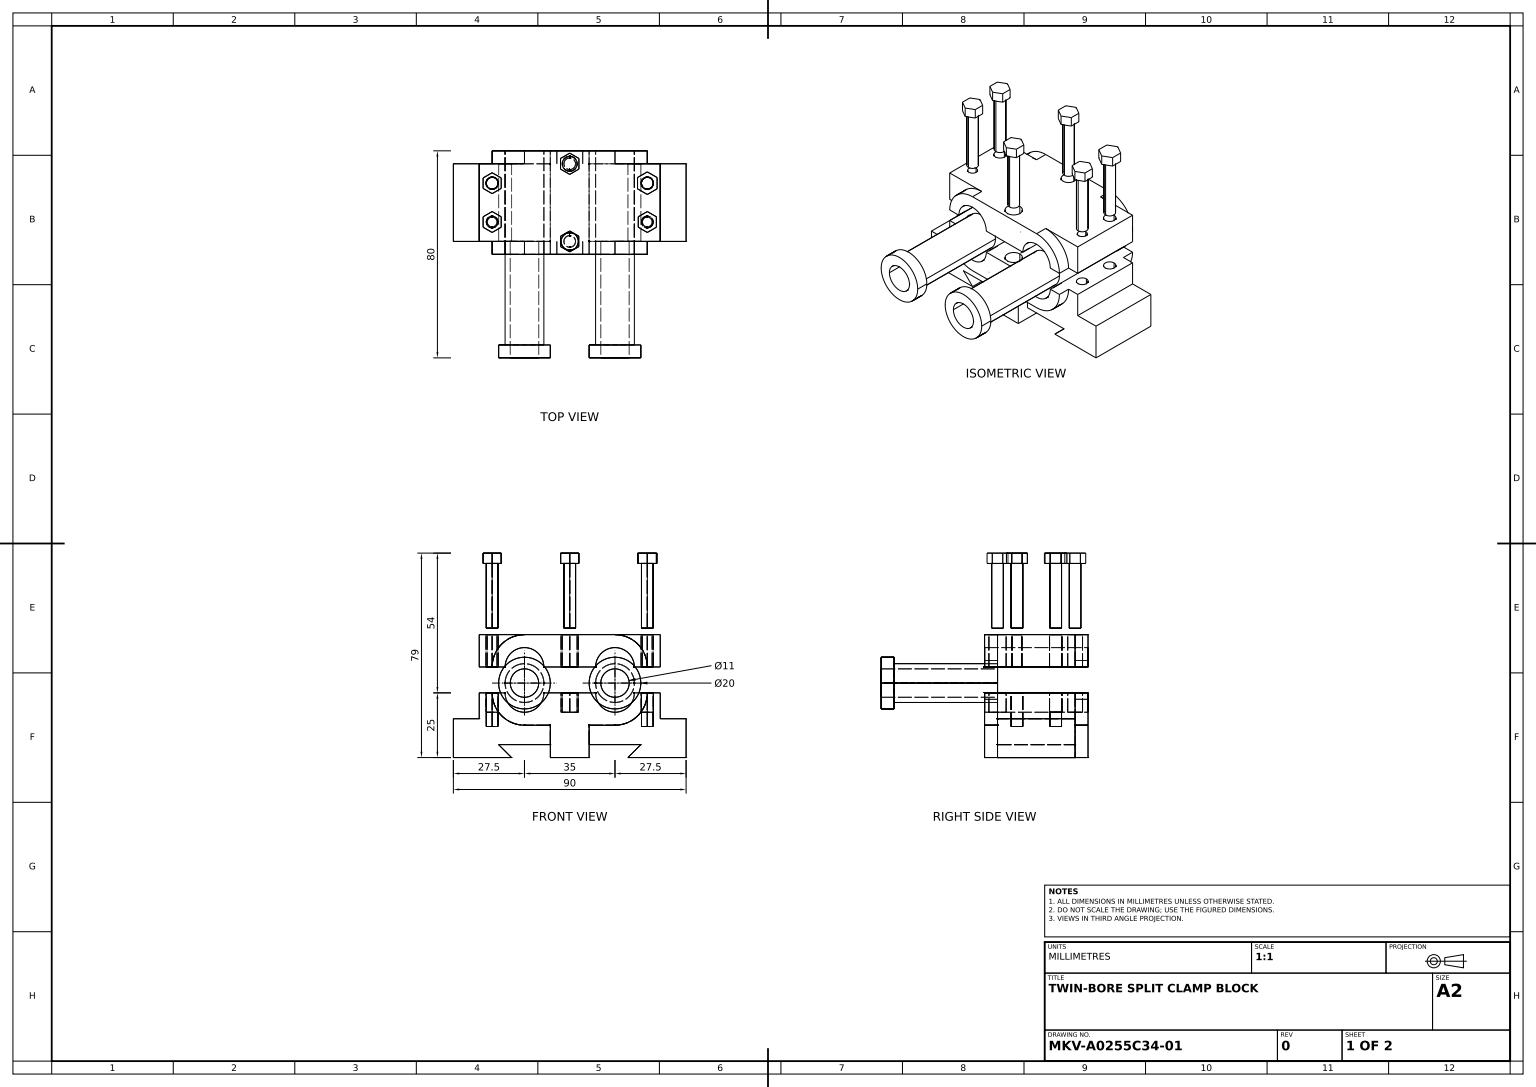
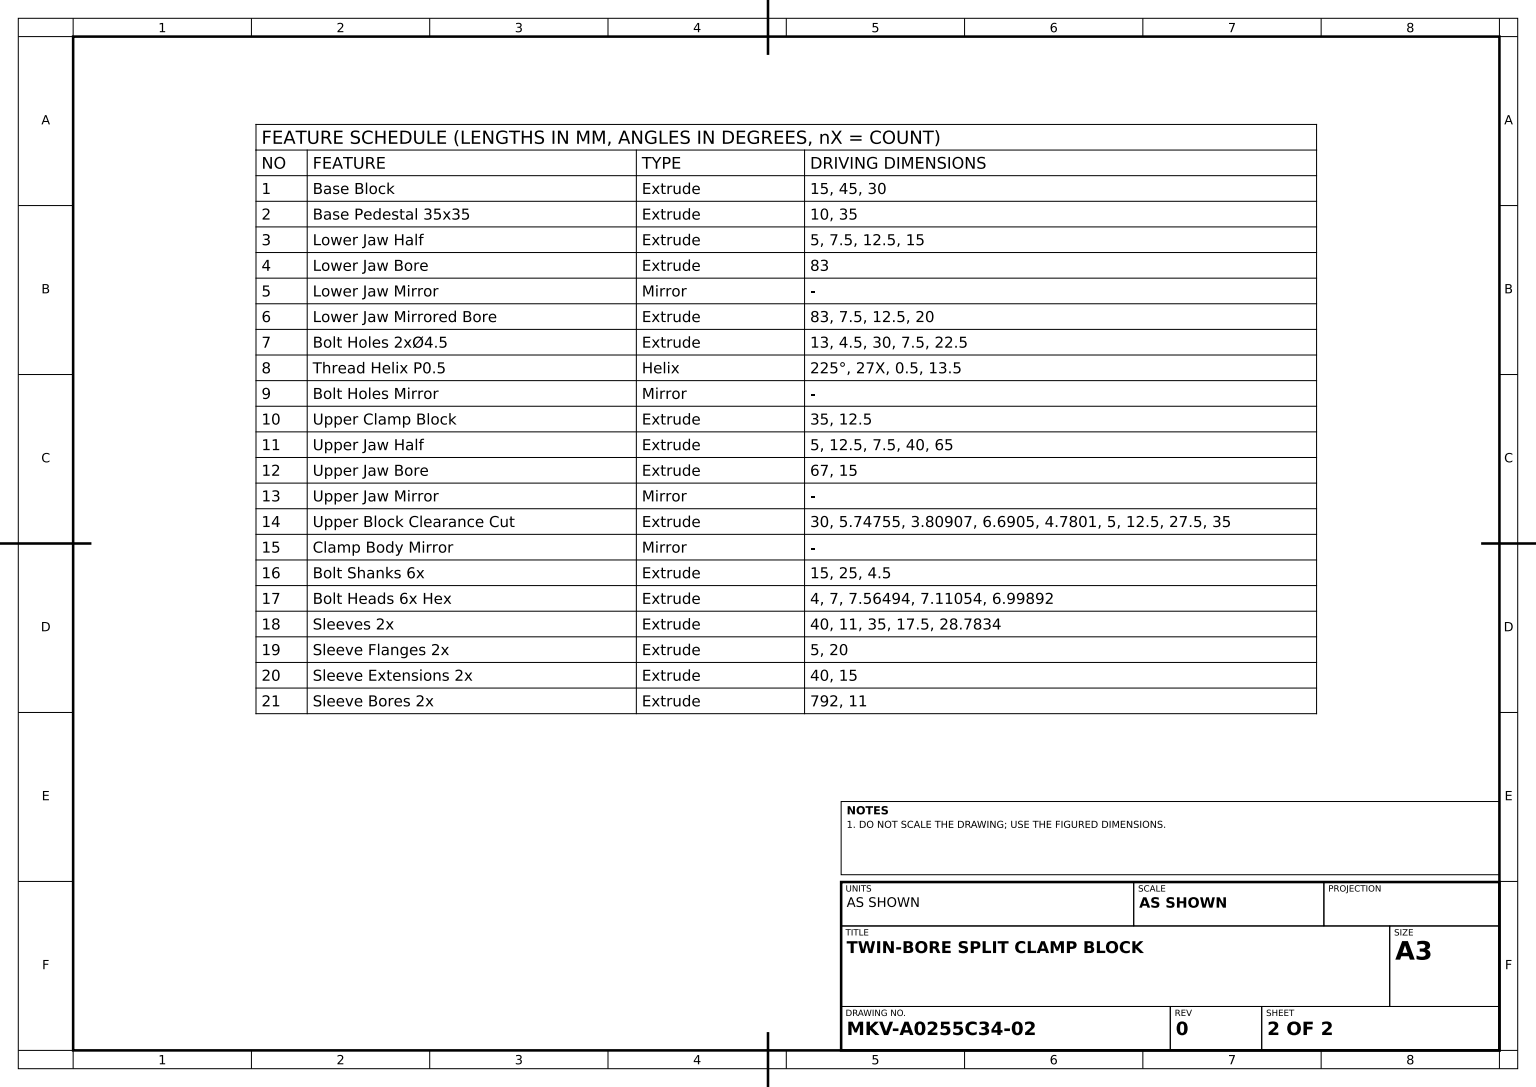
solid
v1 (-7.5,0,5)
v2 (-7.5,12.5,5)
e1 v1 v2 LINE
v3 (-7.5,12.5,0)
e2 v2 v3 LINE
v4 (-7.5,5,0)
e3 v4 v3 LINE
v5 (-7.5,5,-30)
e4 v4 v5 LINE
v6 (-7.5,12.5,-30)
e5 v5 v6 LINE
v7 (-7.5,12.5,-35)
e6 v7 v6 LINE
v8 (-7.5,0,-35)
e7 v8 v7 LINE
e8 v1 v8 LINE
face PLANE(AX(P(-7.5,0,5),D(-1,0,0),D(0,0,1))) [e1 e2 -e3 e4 e5 -e6 -e7 -e8]
v9 (35,15,0)
v10 (35,15,-30)
e9 v9 v10 LINE
v11 (35,25,-30)
e10 v11 v10 LINE
v12 (35,25,0)
e11 v12 v11 LINE
e12 v12 v9 LINE
face PLANE(AX(P(35,25,-30),D(-1,0,0),D(0,0,1))) rev [e9 -e10 -e11 e12]
v13 (-30,25,-20.109948)
v14 (-30,25,-24.890052)
e13 v13 v14 CIRCLE(AX(P(-30,25,-22.5),D(0,1,0),D(0,0,-1)),2.390052)
e14 v14 v13 CIRCLE(AX(P(-30,25,-22.5),D(0,1,0),D(0,0,-1)),2.390052)
v15 (-30,25,-9.75)
v16 (-30,25,-5.25)
e15 v15 v16 CIRCLE(AX(P(-30,25,-7.5),D(0,-1,0),D(0,0,1)),2.25)
e16 v16 v15 CIRCLE(AX(P(-30,25,-7.5),D(0,-1,0),D(0,0,1)),2.25)
v17 (-35,25,0)
v18 (-30,25,0)
e17 v17 v18 LINE
v19 (-30,25,5)
e18 v19 v18 LINE
v20 (-25,25,5)
e19 v20 v19 LINE
v21 (-25,25,-35)
e20 v20 v21 LINE
v22 (-30,25,-35)
e21 v21 v22 LINE
v23 (-30,25,-30)
e22 v22 v23 LINE
v24 (-35,25,-30)
e23 v23 v24 LINE
e24 v24 v17 LINE
face PLANE(AX(P(0,25,0),D(0,-1,0),D(0,0,-1))) rev [-e13 -e14] [e15 e16] [e17 -e18 -e19 e20 e21 e22 e23 e24]
v25 (30,25,-20.109948)
v26 (30,25,-24.890052)
e25 v25 v26 CIRCLE(AX(P(30,25,-22.5),D(0,-1,0),D(0,0,-1)),2.390052)
v27 (30,17.5,-20.109948)
e26 v27 v25 LINE
v28 (30,17.5,-24.890052)
e27 v28 v27 CIRCLE(AX(P(30,17.5,-22.5),D(0,1,0),D(0,0,1)),2.390052)
e28 v28 v26 LINE
face CYL(AX(P(30,17.5,-22.5),D(0,1,0),D(0,0,1)),2.390052) rev [-e25 -e26 -e27 e28]
v29 (0,17.5,3.345252)
v30 (0,25,3.345252)
e29 v29 v30 LINE
v31 (0,25,-3.345252)
e30 v31 v30 CIRCLE(AX(P(0,25,0),D(0,-1,0),D(0,0,-1)),3.345252)
v32 (0,17.5,-3.345252)
e31 v32 v31 LINE
e32 v29 v32 CIRCLE(AX(P(0,17.5,0),D(0,1,0),D(0,0,1)),3.345252)
face CYL(AX(P(0,17.5,0),D(0,1,0),D(0,0,1)),3.345252) rev [e29 -e30 -e31 -e32]
v33 (0,17.5,-32.873773)
v34 (0,25,-32.873773)
e33 v33 v34 LINE
v35 (0,17.5,-27.126227)
e34 v35 v33 CIRCLE(AX(P(0,17.5,-30),D(0,1,0),D(0,0,1)),2.873773)
v36 (0,25,-27.126227)
e35 v35 v36 LINE
e36 v34 v36 CIRCLE(AX(P(0,25,-30),D(0,-1,0),D(0,0,-1)),2.873773)
face CYL(AX(P(0,17.5,-30),D(0,1,0),D(0,0,1)),2.873773) rev [-e33 -e34 e35 -e36]
e37 v32 v29 CIRCLE(AX(P(0,17.5,0),D(0,1,0),D(0,0,1)),3.345252)
e38 v30 v31 CIRCLE(AX(P(0,25,0),D(0,-1,0),D(0,0,-1)),3.345252)
face CYL(AX(P(0,17.5,0),D(0,1,0),D(0,0,1)),3.345252) rev [-e37 e31 -e38 -e29]
v37 (-30,12,-5.25)
v38 (-30,12,-9.75)
e39 v37 v38 CIRCLE(AX(P(-30,12,-7.5),D(0,-1,0),D(0,0,1)),2.25)
e40 v38 v37 CIRCLE(AX(P(-30,12,-7.5),D(0,-1,0),D(0,0,1)),2.25)
face PLANE(AX(P(-30,12,-7.5),D(0,1,0),D(0,0,1))) [-e39 -e40]
v39 (30,12,-5.25)
v40 (30,25,-5.25)
e41 v39 v40 LINE
v41 (30,12,-9.75)
e42 v41 v39 CIRCLE(AX(P(30,12,-7.5),D(0,1,0),D(0,0,1)),2.25)
v42 (30,25,-9.75)
e43 v41 v42 LINE
e44 v42 v40 CIRCLE(AX(P(30,25,-7.5),D(0,1,0),D(0,0,1)),2.25)
face CYL(AX(P(30,12,-7.5),D(0,1,0),D(0,0,1)),2.25) rev [-e41 -e42 e43 e44]
face PLANE(AX(P(0,17.5,0),D(0,1,0),D(0,0,1))) [e37 e32]
v43 (45,0,-30)
v44 (22.5,0,-30)
e45 v43 v44 LINE
v45 (45,0,0)
e46 v45 v43 LINE
v46 (22.5,0,0)
e47 v46 v45 LINE
e48 v46 v44 LINE
face PLANE(AX(P(0,0,0),D(0,-1,0),D(0,0,-1))) [-e45 -e46 -e47 e48]
v47 (17.5,12.5,-35)
v48 (17.5,12.5,-30)
e49 v47 v48 LINE
v49 (30,25,-35)
e50 v47 v49 CIRCLE(AX(P(17.5,25,-35),D(0,0,1),D(1,0,0)),12.5)
v50 (30,25,-30)
e51 v49 v50 LINE
e52 v48 v50 CIRCLE(AX(P(17.5,25,-30),D(0,0,1),D(1,0,0)),12.5)
face CYL(AX(P(17.5,25,-35),D(0,0,1),D(1,0,0)),12.5) [-e49 e50 e51 -e52]
v51 (-17.5,12.5,0)
e53 v3 v51 LINE
v52 (-17.5,12.5,5)
e54 v2 v52 LINE
e55 v52 v51 LINE
face PLANE(AX(P(0,12.5,5),D(0,-1,0),D(0,0,-1))) [-e53 -e2 e54 e55]
v53 (7.5,0,-35)
e56 v8 v53 LINE
v54 (7.5,0,5)
e57 v54 v53 LINE
e58 v1 v54 LINE
face PLANE(AX(P(0,0,0),D(0,-1,0),D(0,0,-1))) [e8 e56 -e57 -e58]
v55 (30,12,-20.25)
v56 (30,12,-24.75)
e59 v55 v56 CIRCLE(AX(P(30,12,-22.5),D(0,1,0),D(0,0,1)),2.25)
v57 (30,17.5,-20.25)
e60 v55 v57 LINE
v58 (30,17.5,-24.75)
e61 v58 v57 CIRCLE(AX(P(30,17.5,-22.5),D(0,-1,0),D(0,0,1)),2.25)
e62 v56 v58 LINE
face CYL(AX(P(30,12,-22.5),D(0,1,0),D(0,0,1)),2.25) rev [-e59 e60 -e61 -e62]
v59 (10,25,5)
v60 (10,25,-35)
e63 v59 v60 LINE
v61 (25,25,5)
e64 v59 v61 CIRCLE(AX(P(17.5,25,5),D(0,0,1),D(1,0,0)),7.5)
v62 (25,25,-35)
e65 v61 v62 LINE
e66 v60 v62 CIRCLE(AX(P(17.5,25,-35),D(0,0,1),D(1,0,0)),7.5)
face CYL(AX(P(17.5,25,5),D(0,0,-1),D(-1,0,0)),7.5) rev [-e63 e64 e65 -e66]
e67 v27 v28 CIRCLE(AX(P(30,17.5,-22.5),D(0,1,0),D(0,0,1)),2.390052)
e68 v57 v58 CIRCLE(AX(P(30,17.5,-22.5),D(0,-1,0),D(0,0,1)),2.25)
face PLANE(AX(P(30,17.5,-22.5),D(0,1,0),D(0,0,1))) [e27 e67] [e61 e68]
v63 (30,25,0)
e69 v63 v12 LINE
e70 v11 v50 LINE
e71 v49 v62 LINE
v64 (30,25,5)
e72 v64 v61 LINE
e73 v64 v63 LINE
e74 v40 v42 CIRCLE(AX(P(30,25,-7.5),D(0,1,0),D(0,0,1)),2.25)
e75 v26 v25 CIRCLE(AX(P(30,25,-22.5),D(0,-1,0),D(0,0,-1)),2.390052)
face PLANE(AX(P(0,25,0),D(0,-1,0),D(0,0,-1))) rev [e69 e11 e70 -e51 e71 -e65 -e72 e73] [-e44 -e74] [e25 e75]
e76 v56 v55 CIRCLE(AX(P(30,12,-22.5),D(0,1,0),D(0,0,1)),2.25)
face PLANE(AX(P(30,12,-22.5),D(0,1,0),D(0,0,1))) [e76 e59]
e77 v36 v34 CIRCLE(AX(P(0,25,-30),D(0,-1,0),D(0,0,-1)),2.873773)
e78 v33 v35 CIRCLE(AX(P(0,17.5,-30),D(0,1,0),D(0,0,1)),2.873773)
face CYL(AX(P(0,17.5,-30),D(0,1,0),D(0,0,1)),2.873773) rev [e33 -e77 -e35 -e78]
e79 v38 v15 LINE
e80 v37 v16 LINE
face CYL(AX(P(-30,12,-7.5),D(0,1,0),D(0,0,1)),2.25) rev [-e15 -e79 e40 e80]
v65 (7.5,12.5,-35)
e81 v65 v47 LINE
v66 (7.5,12.5,-30)
e82 v66 v48 LINE
e83 v65 v66 LINE
face PLANE(AX(P(0,12.5,-35),D(0,-1,0),D(0,0,-1))) [e81 e49 -e82 -e83]
v67 (7.5,12.5,5)
v68 (7.5,12.5,0)
e84 v67 v68 LINE
e85 v54 v67 LINE
e86 v53 v65 LINE
v69 (7.5,5,-30)
e87 v69 v66 LINE
v70 (7.5,5,0)
e88 v70 v69 LINE
e89 v70 v68 LINE
face PLANE(AX(P(7.5,0,5),D(-1,0,0),D(0,0,1))) rev [-e84 -e85 e57 e86 e83 -e87 -e88 e89]
face CYL(AX(P(30,17.5,-22.5),D(0,1,0),D(0,0,1)),2.390052) rev [e26 -e75 -e28 -e67]
v71 (-10,25,-35)
e90 v21 v71 CIRCLE(AX(P(-17.5,25,-35),D(0,0,1),D(1,0,0)),7.5)
v72 (-10,25,5)
e91 v20 v72 CIRCLE(AX(P(-17.5,25,5),D(0,0,1),D(1,0,0)),7.5)
e92 v72 v71 LINE
face CYL(AX(P(-17.5,25,5),D(0,0,-1),D(-1,0,0)),7.5) rev [-e90 -e20 e91 e92]
v73 (-45,0,-30)
v74 (-45,0,0)
e93 v73 v74 LINE
v75 (-45,15,0)
e94 v75 v74 LINE
v76 (-45,15,-30)
e95 v76 v75 LINE
e96 v76 v73 LINE
face PLANE(AX(P(-45,15,0),D(1,0,0),D(0,0,-1))) rev [e93 -e94 -e95 e96]
e97 v59 v72 LINE
e98 v60 v71 LINE
face PLANE(AX(P(0,25,0),D(0,-1,0),D(0,0,-1))) rev [e36 e77] [-e92 -e97 e63 e98] [e30 e38]
v77 (-30,17.5,-24.890052)
v78 (-30,17.5,-20.109948)
e99 v77 v78 CIRCLE(AX(P(-30,17.5,-22.5),D(0,-1,0),D(0,0,1)),2.390052)
e100 v78 v13 LINE
e101 v77 v14 LINE
face CYL(AX(P(-30,17.5,-22.5),D(0,1,0),D(0,0,1)),2.390052) rev [e99 e100 e13 -e101]
v79 (17.5,12.5,5)
e102 v67 v79 LINE
e103 v79 v64 CIRCLE(AX(P(17.5,25,5),D(0,0,1),D(1,0,0)),12.5)
e104 v19 v52 CIRCLE(AX(P(-17.5,25,5),D(0,0,1),D(1,0,0)),12.5)
face PLANE(AX(P(0,0,5),D(0,0,1),D(1,0,0))) [e58 e85 e102 e103 e72 -e64 e97 -e91 e19 e104 -e54 -e1]
face PLANE(AX(P(0,17.5,-30),D(0,1,0),D(0,0,1))) [e78 e34]
e105 v18 v51 CIRCLE(AX(P(-17.5,25,0),D(0,0,1),D(1,0,0)),12.5)
face CYL(AX(P(-17.5,25,5),D(0,0,-1),D(-1,0,0)),12.5) [-e55 -e104 e18 e105]
v80 (45,15,-30)
e106 v80 v43 LINE
v81 (45,15,0)
e107 v81 v80 LINE
e108 v81 v45 LINE
face PLANE(AX(P(45,15,-30),D(-1,0,0),D(0,0,1))) rev [e46 -e106 -e107 e108]
v82 (-30,12,-24.75)
v83 (-30,12,-20.25)
e109 v82 v83 CIRCLE(AX(P(-30,12,-22.5),D(0,-1,0),D(0,0,1)),2.25)
e110 v83 v82 CIRCLE(AX(P(-30,12,-22.5),D(0,-1,0),D(0,0,1)),2.25)
face PLANE(AX(P(-30,12,-22.5),D(0,1,0),D(0,0,1))) [-e109 -e110]
v84 (27.5,5,-30)
e111 v84 v44 LINE
v85 (27.5,5,0)
e112 v85 v46 LINE
e113 v85 v84 LINE
face PLANE(AX(P(11.25,-11.25,53),D(0.707106781,-0.707106781,0),D(0.707106781,0.707106781,0))) rev [e111 -e48 -e112 e113]
v86 (-35,15,0)
e114 v17 v86 LINE
e115 v75 v86 LINE
v87 (-22.5,0,0)
e116 v74 v87 LINE
v88 (-27.5,5,0)
e117 v88 v87 LINE
e118 v4 v88 LINE
face PLANE(AX(P(0,15,0),D(0,0,-1),D(-1,0,0))) rev [-e105 -e17 e114 -e115 e94 e116 -e117 -e118 e3 e53]
e119 v84 v69 LINE
e120 v80 v10 LINE
face PLANE(AX(P(-45,15,-30),D(0,0,1),D(1,0,0))) rev [e119 e87 e82 e52 -e70 e10 -e120 e106 e45 -e111]
e121 v78 v77 CIRCLE(AX(P(-30,17.5,-22.5),D(0,-1,0),D(0,0,1)),2.390052)
face CYL(AX(P(-30,17.5,-22.5),D(0,1,0),D(0,0,1)),2.390052) rev [-e100 e121 e101 e14]
v89 (-22.5,0,-30)
e122 v89 v73 LINE
e123 v87 v89 LINE
face PLANE(AX(P(0,0,0),D(0,-1,0),D(0,0,-1))) [-e116 -e93 -e122 -e123]
v90 (-17.5,12.5,-35)
e124 v22 v90 CIRCLE(AX(P(-17.5,25,-35),D(0,0,1),D(1,0,0)),12.5)
v91 (-17.5,12.5,-30)
e125 v90 v91 LINE
e126 v23 v91 CIRCLE(AX(P(-17.5,25,-30),D(0,0,1),D(1,0,0)),12.5)
face CYL(AX(P(-17.5,25,-35),D(0,0,1),D(1,0,0)),12.5) [-e22 e124 e125 -e126]
v92 (17.5,12.5,0)
e127 v68 v92 LINE
e128 v79 v92 LINE
face PLANE(AX(P(0,12.5,5),D(0,1,0),D(0,0,1))) rev [-e102 e84 e127 -e128]
v93 (-35,15,-30)
e129 v24 v93 LINE
e130 v6 v91 LINE
v94 (-27.5,5,-30)
e131 v5 v94 LINE
e132 v94 v89 LINE
e133 v93 v76 LINE
face PLANE(AX(P(-45,15,-30),D(0,0,1),D(1,0,0))) rev [-e129 -e23 e126 -e130 -e5 e131 e132 e122 -e96 -e133]
e134 v7 v90 LINE
face PLANE(AX(P(0,0,-35),D(0,0,-1),D(1,0,0))) [-e86 -e56 e7 e134 -e124 -e21 e90 -e98 e66 -e71 -e50 -e81]
v95 (-30,17.5,-20.25)
e135 v83 v95 LINE
v96 (-30,17.5,-24.75)
e136 v95 v96 CIRCLE(AX(P(-30,17.5,-22.5),D(0,1,0),D(0,0,1)),2.25)
e137 v82 v96 LINE
face CYL(AX(P(-30,12,-22.5),D(0,1,0),D(0,0,1)),2.25) rev [e135 e136 -e137 e109]
e138 v93 v86 LINE
face PLANE(AX(P(0,15,0),D(0,-1,0),D(0,0,-1))) rev [e115 -e138 e133 e95]
e139 v39 v41 CIRCLE(AX(P(30,12,-7.5),D(0,1,0),D(0,0,1)),2.25)
face PLANE(AX(P(30,12,-7.5),D(0,1,0),D(0,0,1))) [e42 e139]
face CYL(AX(P(30,12,-22.5),D(0,1,0),D(0,0,1)),2.25) rev [-e68 -e60 -e76 e62]
e140 v92 v63 CIRCLE(AX(P(17.5,25,0),D(0,0,1),D(1,0,0)),12.5)
face CYL(AX(P(17.5,25,5),D(0,0,-1),D(-1,0,0)),12.5) [-e103 e128 e140 -e73]
e141 v85 v70 LINE
e142 v9 v81 LINE
face PLANE(AX(P(0,15,0),D(0,0,-1),D(-1,0,0))) rev [-e141 e112 e47 -e108 -e142 -e12 -e69 -e140 -e127 -e89]
e143 v96 v95 CIRCLE(AX(P(-30,17.5,-22.5),D(0,1,0),D(0,0,1)),2.25)
face CYL(AX(P(-30,12,-22.5),D(0,1,0),D(0,0,1)),2.25) rev [e110 e137 e143 -e135]
face PLANE(AX(P(0,5,53),D(0,-1,0),D(1,0,0))) [e88 -e119 -e113 e141]
e144 v88 v94 LINE
face PLANE(AX(P(-11.25,-11.25,53),D(0.707106781,0.707106781,0),D(-0.707106781,0.707106781,0))) [e123 -e132 -e144 e117]
face PLANE(AX(P(0,15,0),D(0,-1,0),D(0,0,-1))) rev [e142 e107 e120 -e9]
face PLANE(AX(P(-30,17.5,-22.5),D(0,1,0),D(0,0,1))) [-e121 -e99] [-e143 -e136]
face PLANE(AX(P(0,12.5,-35),D(0,1,0),D(0,0,1))) rev [-e134 e6 e130 -e125]
face PLANE(AX(P(0,5,53),D(0,-1,0),D(1,0,0))) [e144 -e131 -e4 e118]
face PLANE(AX(P(-35,25,0),D(1,0,0),D(0,0,-1))) rev [-e114 -e24 e129 e138]
face CYL(AX(P(30,12,-7.5),D(0,1,0),D(0,0,1)),2.25) rev [e74 -e43 -e139 e41]
face CYL(AX(P(-30,12,-7.5),D(0,1,0),D(0,0,1)),2.25) rev [-e80 e39 e79 -e16]
solid
v97 (33.78247,79,-24.68381)
v98 (33.78247,75,-24.68381)
e145 v97 v98 LINE
v99 (33.78247,79,-20.31619)
e146 v99 v97 LINE
v100 (33.78247,75,-20.31619)
e147 v99 v100 LINE
e148 v100 v98 LINE
face PLANE(AX(P(33.78247,79,-20.31619),D(-1,0,0),D(0,0,1))) rev [-e145 -e146 e147 e148]
v101 (30,75,-26.86762)
e149 v98 v101 LINE
v102 (30,79,-26.86762)
e150 v102 v101 LINE
e151 v97 v102 LINE
face PLANE(AX(P(33.78247,79,-24.68381),D(-0.5,0,0.866025404),D(0.866025404,0,0.5))) rev [e149 -e150 -e151 e145]
v103 (26.21753,79,-24.68381)
e152 v102 v103 LINE
v104 (26.21753,79,-20.31619)
e153 v103 v104 LINE
v105 (30,79,-18.13238)
e154 v104 v105 LINE
e155 v105 v99 LINE
face PLANE(AX(P(0,79,0),D(0,1,0),D(0,0,1))) [e151 e152 e153 e154 e155 e146]
v106 (26.21753,75,-24.68381)
e156 v103 v106 LINE
v107 (26.21753,75,-20.31619)
e157 v106 v107 LINE
e158 v104 v107 LINE
face PLANE(AX(P(26.21753,79,-24.68381),D(1,0,0),D(0,0,-1))) rev [e156 e157 -e158 -e153]
v108 (30,75,-20.25)
v109 (30,50,-20.25)
e159 v108 v109 LINE
v110 (30,50,-24.75)
e160 v109 v110 CIRCLE(AX(P(30,50,-22.5),D(0,1,0),D(0,0,1)),2.25)
v111 (30,75,-24.75)
e161 v111 v110 LINE
e162 v108 v111 CIRCLE(AX(P(30,75,-22.5),D(0,1,0),D(0,0,1)),2.25)
face CYL(AX(P(30,75,-22.5),D(0,-1,0),D(0,0,-1)),2.25) [e159 e160 -e161 -e162]
e163 v101 v106 LINE
v112 (30,75,-18.13238)
e164 v112 v100 LINE
e165 v107 v112 LINE
e166 v111 v108 CIRCLE(AX(P(30,75,-22.5),D(0,1,0),D(0,0,1)),2.25)
face PLANE(AX(P(0,75,0),D(0,1,0),D(0,0,1))) rev [-e163 -e149 -e148 -e164 -e165 -e157] [e162 e166]
e167 v110 v109 CIRCLE(AX(P(30,50,-22.5),D(0,1,0),D(0,0,1)),2.25)
face PLANE(AX(P(30,50,-22.5),D(0,1,0),D(0,0,1))) rev [-e160 -e167]
face CYL(AX(P(30,75,-22.5),D(0,-1,0),D(0,0,-1)),2.25) [e161 e167 -e159 -e166]
e168 v105 v112 LINE
face PLANE(AX(P(26.21753,79,-20.31619),D(0.5,0,-0.866025404),D(-0.866025404,0,-0.5))) rev [-e168 -e154 e158 e165]
face PLANE(AX(P(30,79,-18.13238),D(-0.5,0,-0.866025404),D(-0.866025404,0,0.5))) rev [-e147 -e155 e168 e164]
face PLANE(AX(P(30,79,-26.86762),D(0.5,0,0.866025404),D(0.866025404,0,-0.5))) rev [e150 e163 -e156 -e152]
solid
v113 (-30,35,-20.109948)
v114 (-30,47.5,-20.109948)
e169 v113 v114 LINE
v115 (-30,47.5,-24.890052)
e170 v115 v114 CIRCLE(AX(P(-30,47.5,-22.5),D(0,-1,0),D(0,0,1)),2.390052)
v116 (-30,35,-24.890052)
e171 v116 v115 LINE
e172 v113 v116 CIRCLE(AX(P(-30,35,-22.5),D(0,1,0),D(0,0,-1)),2.390052)
face CYL(AX(P(-30,17.5,-22.5),D(0,1,0),D(0,0,1)),2.390052) rev [e169 -e170 -e171 -e172]
v117 (-30,35,5)
v118 (-30,35,0)
e173 v117 v118 LINE
v119 (-17.5,47.5,5)
e174 v119 v117 CIRCLE(AX(P(-17.5,35,5),D(0,0,1),D(1,0,0)),12.5)
v120 (-17.5,47.5,0)
e175 v119 v120 LINE
e176 v120 v118 CIRCLE(AX(P(-17.5,35,0),D(0,0,1),D(1,0,0)),12.5)
face CYL(AX(P(-17.5,35,5),D(0,0,-1),D(-1,0,0)),12.5) [-e173 -e174 e175 e176]
v121 (-35,47.5,0)
v122 (-35,35,0)
e177 v121 v122 LINE
v123 (-35,47.5,-30)
e178 v123 v121 LINE
v124 (-35,35,-30)
e179 v123 v124 LINE
e180 v124 v122 LINE
face PLANE(AX(P(-35,47.5,0),D(1,0,0),D(0,0,-1))) rev [-e177 -e178 e179 e180]
v125 (35,47.5,0)
v126 (35,35,0)
e181 v125 v126 LINE
v127 (17.5,47.5,0)
e182 v127 v125 LINE
v128 (30,35,0)
e183 v128 v127 CIRCLE(AX(P(17.5,35,0),D(0,0,1),D(1,0,0)),12.5)
e184 v128 v126 LINE
face PLANE(AX(P(35,47.5,0),D(0,0,-1),D(-1,0,0))) rev [-e181 -e182 -e183 e184]
e185 v121 v120 LINE
e186 v122 v118 LINE
face PLANE(AX(P(35,47.5,0),D(0,0,-1),D(-1,0,0))) rev [-e185 e177 e186 -e176]
v129 (0,35,-32.873773)
v130 (0,47.5,-32.873773)
e187 v129 v130 LINE
v131 (0,47.5,-27.126227)
e188 v130 v131 CIRCLE(AX(P(0,47.5,-30),D(0,1,0),D(0,0,1)),2.873773)
v132 (0,35,-27.126227)
e189 v132 v131 LINE
e190 v132 v129 CIRCLE(AX(P(0,35,-30),D(0,-1,0),D(0,0,-1)),2.873773)
face CYL(AX(P(0,17.5,-30),D(0,1,0),D(0,0,1)),2.873773) rev [e187 e188 -e189 e190]
v133 (30,47.5,-5.595463)
v134 (30,47.5,-9.404537)
e191 v133 v134 CIRCLE(AX(P(30,47.5,-7.5),D(0,1,0),D(0,0,1)),1.904537)
e192 v134 v133 CIRCLE(AX(P(30,47.5,-7.5),D(0,1,0),D(0,0,1)),1.904537)
v135 (17.5,47.5,-35)
v136 (-17.5,47.5,-35)
e193 v135 v136 LINE
v137 (-17.5,47.5,-30)
e194 v136 v137 LINE
e195 v137 v123 LINE
v138 (17.5,47.5,5)
e196 v138 v119 LINE
e197 v138 v127 LINE
v139 (35,47.5,-30)
e198 v125 v139 LINE
v140 (17.5,47.5,-30)
e199 v139 v140 LINE
e200 v135 v140 LINE
v141 (-30,47.5,-5.595463)
v142 (-30,47.5,-9.404537)
e201 v141 v142 CIRCLE(AX(P(-30,47.5,-7.5),D(0,-1,0),D(0,0,1)),1.904537)
e202 v142 v141 CIRCLE(AX(P(-30,47.5,-7.5),D(0,-1,0),D(0,0,1)),1.904537)
v143 (30,47.5,-20.109948)
v144 (30,47.5,-24.890052)
e203 v143 v144 CIRCLE(AX(P(30,47.5,-22.5),D(0,1,0),D(0,0,1)),2.390052)
e204 v144 v143 CIRCLE(AX(P(30,47.5,-22.5),D(0,1,0),D(0,0,1)),2.390052)
v145 (0,47.5,3.345252)
v146 (0,47.5,-3.345252)
e205 v145 v146 CIRCLE(AX(P(0,47.5,0),D(0,1,0),D(0,0,1)),3.345252)
e206 v146 v145 CIRCLE(AX(P(0,47.5,0),D(0,1,0),D(0,0,1)),3.345252)
e207 v114 v115 CIRCLE(AX(P(-30,47.5,-22.5),D(0,-1,0),D(0,0,1)),2.390052)
e208 v131 v130 CIRCLE(AX(P(0,47.5,-30),D(0,1,0),D(0,0,1)),2.873773)
face PLANE(AX(P(0,47.5,0),D(0,-1,0),D(0,0,-1))) rev [-e191 -e192] [e193 e194 e195 e178 e185 -e175 -e196 e197 e182 e198 e199 -e200] [e201 e202] [-e203 -e204] [-e205 -e206] [e170 e207] [-e208 -e188]
v147 (-30,35,-5.595463)
v148 (-30,35,-9.404537)
e209 v147 v148 CIRCLE(AX(P(-30,35,-7.5),D(0,1,0),D(0,0,-1)),1.904537)
e210 v148 v147 CIRCLE(AX(P(-30,35,-7.5),D(0,1,0),D(0,0,-1)),1.904537)
v149 (-30,35,-35)
v150 (-25,35,-35)
e211 v149 v150 LINE
v151 (-25,35,5)
e212 v151 v150 LINE
e213 v117 v151 LINE
v152 (-30,35,-30)
e214 v152 v124 LINE
e215 v149 v152 LINE
e216 v116 v113 CIRCLE(AX(P(-30,35,-22.5),D(0,1,0),D(0,0,-1)),2.390052)
face PLANE(AX(P(0,35,0),D(0,-1,0),D(0,0,-1))) [e209 e210] [e211 -e212 -e213 e173 -e186 -e180 -e214 -e215] [e172 e216]
v153 (30,35,-35)
e217 v153 v135 CIRCLE(AX(P(17.5,35,-35),D(0,0,1),D(1,0,0)),12.5)
v154 (30,35,-30)
e218 v154 v140 CIRCLE(AX(P(17.5,35,-30),D(0,0,1),D(1,0,0)),12.5)
e219 v153 v154 LINE
face CYL(AX(P(17.5,35,-35),D(0,0,1),D(1,0,0)),12.5) [e217 e200 -e218 -e219]
v155 (30,35,-9.404537)
e220 v155 v134 LINE
v156 (30,35,-5.595463)
e221 v155 v156 CIRCLE(AX(P(30,35,-7.5),D(0,-1,0),D(0,0,-1)),1.904537)
e222 v156 v133 LINE
face CYL(AX(P(30,17.5,-7.5),D(0,1,0),D(0,0,1)),1.904537) rev [-e220 e221 e222 e191]
v157 (30,35,-24.890052)
v158 (30,35,-20.109948)
e223 v157 v158 CIRCLE(AX(P(30,35,-22.5),D(0,-1,0),D(0,0,-1)),2.390052)
e224 v158 v157 CIRCLE(AX(P(30,35,-22.5),D(0,-1,0),D(0,0,-1)),2.390052)
e225 v156 v155 CIRCLE(AX(P(30,35,-7.5),D(0,-1,0),D(0,0,-1)),1.904537)
v159 (35,35,-30)
e226 v126 v159 LINE
v160 (30,35,5)
e227 v160 v128 LINE
v161 (25,35,5)
e228 v161 v160 LINE
v162 (25,35,-35)
e229 v161 v162 LINE
e230 v162 v153 LINE
e231 v159 v154 LINE
face PLANE(AX(P(0,35,0),D(0,-1,0),D(0,0,-1))) [-e223 -e224] [-e221 -e225] [-e226 -e184 -e227 -e228 e229 e230 e219 -e231]
e232 v158 v143 LINE
e233 v157 v144 LINE
face CYL(AX(P(30,17.5,-22.5),D(0,1,0),D(0,0,1)),2.390052) rev [e204 -e232 e224 e233]
v163 (10,35,5)
e234 v161 v163 CIRCLE(AX(P(17.5,35,5),D(0,0,1),D(1,0,0)),7.5)
v164 (10,35,-35)
e235 v163 v164 LINE
e236 v162 v164 CIRCLE(AX(P(17.5,35,-35),D(0,0,1),D(1,0,0)),7.5)
face CYL(AX(P(17.5,35,5),D(0,0,-1),D(-1,0,0)),7.5) rev [-e229 e234 e235 -e236]
face CYL(AX(P(-30,17.5,-22.5),D(0,1,0),D(0,0,1)),2.390052) rev [-e169 -e216 e171 -e207]
e237 v148 v142 LINE
e238 v147 v141 LINE
face CYL(AX(P(-30,17.5,-7.5),D(0,1,0),D(0,0,1)),1.904537) rev [-e202 -e237 -e209 e238]
e239 v137 v152 CIRCLE(AX(P(-17.5,35,-30),D(0,0,1),D(1,0,0)),12.5)
face PLANE(AX(P(-35,47.5,-30),D(0,0,1),D(1,0,0))) rev [e214 -e179 -e195 e239]
face CYL(AX(P(30,17.5,-22.5),D(0,1,0),D(0,0,1)),2.390052) rev [e203 -e233 e223 e232]
v165 (0,35,3.345252)
e240 v165 v145 LINE
v166 (0,35,-3.345252)
e241 v166 v146 LINE
e242 v166 v165 CIRCLE(AX(P(0,35,0),D(0,-1,0),D(0,0,-1)),3.345252)
face CYL(AX(P(0,17.5,0),D(0,1,0),D(0,0,1)),3.345252) rev [e240 e205 -e241 e242]
v167 (-10,35,-35)
e243 v167 v150 CIRCLE(AX(P(-17.5,35,-35),D(0,0,1),D(1,0,0)),7.5)
v168 (-10,35,5)
e244 v168 v167 LINE
e245 v168 v151 CIRCLE(AX(P(-17.5,35,5),D(0,0,1),D(1,0,0)),7.5)
face CYL(AX(P(-17.5,35,5),D(0,0,-1),D(-1,0,0)),7.5) rev [e212 -e243 -e244 e245]
e246 v167 v164 LINE
e247 v168 v163 LINE
e248 v165 v166 CIRCLE(AX(P(0,35,0),D(0,-1,0),D(0,0,-1)),3.345252)
e249 v129 v132 CIRCLE(AX(P(0,35,-30),D(0,-1,0),D(0,0,-1)),2.873773)
face PLANE(AX(P(0,35,0),D(0,-1,0),D(0,0,-1))) [e244 e246 -e235 -e247] [-e248 -e242] [-e249 -e190]
face CYL(AX(P(0,17.5,-30),D(0,1,0),D(0,0,1)),2.873773) rev [e189 e208 -e187 e249]
e250 v136 v149 CIRCLE(AX(P(-17.5,35,-35),D(0,0,1),D(1,0,0)),12.5)
face PLANE(AX(P(0,0,-35),D(0,0,-1),D(1,0,0))) [e243 -e211 -e250 -e193 -e217 -e230 e236 -e246]
e251 v160 v138 CIRCLE(AX(P(17.5,35,5),D(0,0,1),D(1,0,0)),12.5)
face CYL(AX(P(17.5,35,5),D(0,0,-1),D(-1,0,0)),12.5) [-e251 e227 e183 -e197]
face CYL(AX(P(-17.5,35,-35),D(0,0,1),D(1,0,0)),12.5) [e250 e215 -e239 -e194]
e252 v139 v159 LINE
face PLANE(AX(P(-35,47.5,-30),D(0,0,1),D(1,0,0))) rev [-e199 e252 e231 e218]
face CYL(AX(P(0,17.5,0),D(0,1,0),D(0,0,1)),3.345252) rev [e206 -e240 e248 e241]
face PLANE(AX(P(0,0,5),D(0,0,1),D(1,0,0))) [e247 -e234 e228 e251 e196 e174 e213 -e245]
face PLANE(AX(P(35,47.5,-30),D(-1,0,0),D(0,0,1))) rev [-e252 -e198 e181 e226]
face CYL(AX(P(-30,17.5,-7.5),D(0,1,0),D(0,0,1)),1.904537) rev [e237 -e201 -e238 -e210]
face CYL(AX(P(30,17.5,-7.5),D(0,1,0),D(0,0,1)),1.904537) rev [e220 e192 -e222 e225]
solid
v169 (-33.5,75,-20.479274)
v170 (-30,75,-18.458548)
e253 v169 v170 LINE
v171 (-33.5,75,-24.520726)
e254 v171 v169 LINE
v172 (-30,75,-26.541452)
e255 v172 v171 LINE
v173 (-26.5,75,-24.520726)
e256 v173 v172 LINE
v174 (-26.5,75,-20.479274)
e257 v174 v173 LINE
e258 v170 v174 LINE
v175 (-30,75,-20.25)
v176 (-30,75,-24.75)
e259 v175 v176 CIRCLE(AX(P(-30,75,-22.5),D(0,1,0),D(0,0,1)),2.25)
e260 v176 v175 CIRCLE(AX(P(-30,75,-22.5),D(0,1,0),D(0,0,1)),2.25)
face PLANE(AX(P(0,75,0),D(0,1,0),D(0,0,1))) rev [-e253 -e254 -e255 -e256 -e257 -e258] [e259 e260]
v177 (-30,79,-26.541452)
e261 v177 v172 LINE
v178 (-33.5,79,-24.520726)
e262 v178 v171 LINE
e263 v177 v178 LINE
face PLANE(AX(P(-30,79,-26.541452),D(0.5,0,0.866025404),D(0.866025404,0,-0.5))) rev [e261 e255 -e262 -e263]
v179 (-33.5,79,-20.479274)
e264 v179 v169 LINE
e265 v178 v179 LINE
face PLANE(AX(P(-33.5,79,-24.520726),D(1,0,0),D(0,0,-1))) rev [-e264 -e265 e262 e254]
v180 (-26.5,79,-20.479274)
v181 (-26.5,79,-24.520726)
e266 v180 v181 LINE
e267 v181 v177 LINE
v182 (-30,79,-18.458548)
e268 v179 v182 LINE
e269 v182 v180 LINE
face PLANE(AX(P(0,79,0),D(0,1,0),D(0,0,1))) [e266 e267 e263 e265 e268 e269]
v183 (-30,50,-24.75)
v184 (-30,50,-20.25)
e270 v183 v184 CIRCLE(AX(P(-30,50,-22.5),D(0,1,0),D(0,0,1)),2.25)
e271 v184 v183 CIRCLE(AX(P(-30,50,-22.5),D(0,1,0),D(0,0,1)),2.25)
face PLANE(AX(P(-30,50,-22.5),D(0,1,0),D(0,0,1))) rev [-e270 -e271]
e272 v175 v184 LINE
e273 v176 v183 LINE
face CYL(AX(P(-30,75,-22.5),D(0,-1,0),D(0,0,-1)),2.25) [-e272 -e260 e273 e270]
face CYL(AX(P(-30,75,-22.5),D(0,-1,0),D(0,0,-1)),2.25) [e272 e271 -e273 -e259]
e274 v182 v170 LINE
e275 v180 v174 LINE
face PLANE(AX(P(-30,79,-18.458548),D(-0.5,0,-0.866025404),D(-0.866025404,0,0.5))) rev [e274 e258 -e275 -e269]
face PLANE(AX(P(-33.5,79,-20.479274),D(0.5,0,-0.866025404),D(-0.866025404,0,-0.5))) rev [-e274 -e268 e264 e253]
e276 v181 v173 LINE
face PLANE(AX(P(-26.5,79,-24.520726),D(-0.5,0,0.866025404),D(0.866025404,0,0.5))) rev [e256 -e261 -e267 e276]
face PLANE(AX(P(-26.5,79,-20.479274),D(-1,0,0),D(0,0,1))) rev [-e276 -e266 e275 e257]
solid
v185 (0,75,-34.105272)
v186 (-3.55527,75,-32.052636)
e277 v185 v186 LINE
v187 (-3.55527,79,-32.052636)
e278 v187 v186 LINE
v188 (0,79,-34.105272)
e279 v188 v187 LINE
e280 v188 v185 LINE
face PLANE(AX(P(0,79,-34.105272),D(0.5,0,0.866025404),D(0.866025404,0,-0.5))) rev [e277 -e278 -e279 e280]
v189 (0,75,-32.25)
v190 (0,50,-32.25)
e281 v189 v190 LINE
v191 (0,75,-27.75)
e282 v191 v189 CIRCLE(AX(P(0,75,-30),D(0,1,0),D(0,0,1)),2.25)
v192 (0,50,-27.75)
e283 v191 v192 LINE
e284 v192 v190 CIRCLE(AX(P(0,50,-30),D(0,1,0),D(0,0,1)),2.25)
face CYL(AX(P(0,75,-30),D(0,-1,0),D(0,0,-1)),2.25) [-e281 -e282 e283 e284]
v193 (3.55527,79,-27.947364)
v194 (3.55527,75,-27.947364)
e285 v193 v194 LINE
v195 (3.55527,75,-32.052636)
e286 v194 v195 LINE
v196 (3.55527,79,-32.052636)
e287 v196 v195 LINE
e288 v193 v196 LINE
face PLANE(AX(P(3.55527,79,-27.947364),D(-1,0,0),D(0,0,1))) rev [e285 e286 -e287 -e288]
v197 (0,75,-25.894728)
e289 v197 v194 LINE
v198 (-3.55527,75,-27.947364)
e290 v198 v197 LINE
e291 v186 v198 LINE
e292 v195 v185 LINE
e293 v189 v191 CIRCLE(AX(P(0,75,-30),D(0,1,0),D(0,0,1)),2.25)
face PLANE(AX(P(0,75,0),D(0,1,0),D(0,0,1))) rev [-e286 -e289 -e290 -e291 -e277 -e292] [e293 e282]
v199 (-3.55527,79,-27.947364)
e294 v187 v199 LINE
e295 v199 v198 LINE
face PLANE(AX(P(-3.55527,79,-32.052636),D(1,0,0),D(0,0,-1))) rev [-e294 e278 e291 -e295]
e296 v190 v192 CIRCLE(AX(P(0,50,-30),D(0,1,0),D(0,0,1)),2.25)
face CYL(AX(P(0,75,-30),D(0,-1,0),D(0,0,-1)),2.25) [-e283 -e293 e281 e296]
v200 (0,79,-25.894728)
e297 v199 v200 LINE
e298 v200 v193 LINE
e299 v196 v188 LINE
face PLANE(AX(P(0,79,0),D(0,1,0),D(0,0,1))) [e279 e294 e297 e298 e288 e299]
face PLANE(AX(P(0,50,-30),D(0,1,0),D(0,0,1))) rev [-e296 -e284]
e300 v200 v197 LINE
face PLANE(AX(P(0,79,-25.894728),D(-0.5,0,-0.866025404),D(-0.866025404,0,0.5))) rev [e300 e289 -e285 -e298]
face PLANE(AX(P(-3.55527,79,-27.947364),D(0.5,0,-0.866025404),D(-0.866025404,0,-0.5))) rev [-e297 e295 e290 -e300]
face PLANE(AX(P(3.55527,79,-32.052636),D(-0.5,0,0.866025404),D(0.866025404,0,0.5))) rev [e287 e292 -e280 -e299]
solid
v201 (0,50,2.25)
v202 (0,50,-2.25)
e301 v201 v202 CIRCLE(AX(P(0,50,0),D(0,1,0),D(0,0,1)),2.25)
e302 v202 v201 CIRCLE(AX(P(0,50,0),D(0,1,0),D(0,0,1)),2.25)
face PLANE(AX(P(0,50,0),D(0,1,0),D(0,0,1))) rev [-e301 -e302]
v203 (-3.5,75,2.020726)
v204 (0,75,4.041452)
e303 v203 v204 LINE
v205 (-3.5,75,-2.020726)
e304 v205 v203 LINE
v206 (0,75,-4.041452)
e305 v206 v205 LINE
v207 (3.5,75,-2.020726)
e306 v207 v206 LINE
v208 (3.5,75,2.020726)
e307 v208 v207 LINE
e308 v204 v208 LINE
v209 (0,75,2.25)
v210 (0,75,-2.25)
e309 v209 v210 CIRCLE(AX(P(0,75,0),D(0,1,0),D(0,0,1)),2.25)
e310 v210 v209 CIRCLE(AX(P(0,75,0),D(0,1,0),D(0,0,1)),2.25)
face PLANE(AX(P(0,75,0),D(0,1,0),D(0,0,1))) rev [-e303 -e304 -e305 -e306 -e307 -e308] [e309 e310]
v211 (3.5,79,2.020726)
e311 v211 v208 LINE
v212 (0,79,4.041452)
e312 v212 v211 LINE
e313 v212 v204 LINE
face PLANE(AX(P(0,79,4.041452),D(-0.5,0,-0.866025404),D(-0.866025404,0,0.5))) rev [-e311 -e312 e313 e308]
e314 v209 v201 LINE
e315 v210 v202 LINE
face CYL(AX(P(0,75,0),D(0,-1,0),D(0,0,-1)),2.25) [e314 e301 -e315 -e309]
face CYL(AX(P(0,75,0),D(0,-1,0),D(0,0,-1)),2.25) [-e310 e315 e302 -e314]
v213 (-3.5,79,2.020726)
e316 v213 v212 LINE
e317 v213 v203 LINE
face PLANE(AX(P(-3.5,79,2.020726),D(0.5,0,-0.866025404),D(-0.866025404,0,-0.5))) rev [-e316 e317 e303 -e313]
v214 (-3.5,79,-2.020726)
e318 v214 v205 LINE
e319 v214 v213 LINE
face PLANE(AX(P(-3.5,79,-2.020726),D(1,0,0),D(0,0,-1))) rev [e318 e304 -e317 -e319]
v215 (3.5,79,-2.020726)
e320 v215 v207 LINE
e321 v211 v215 LINE
face PLANE(AX(P(3.5,79,2.020726),D(-1,0,0),D(0,0,1))) rev [e307 -e320 -e321 e311]
v216 (0,79,-4.041452)
e322 v215 v216 LINE
e323 v216 v214 LINE
face PLANE(AX(P(0,79,0),D(0,1,0),D(0,0,1))) [e316 e312 e321 e322 e323 e319]
e324 v216 v206 LINE
face PLANE(AX(P(3.5,79,-2.020726),D(-0.5,0,0.866025404),D(0.866025404,0,0.5))) rev [e306 -e324 -e322 e320]
face PLANE(AX(P(0,79,-4.041452),D(0.5,0,0.866025404),D(0.866025404,0,-0.5))) rev [e324 e305 -e318 -e323]
solid
v217 (27.5,28.78335,45)
v218 (7.5,28.78335,45)
e325 v217 v218 CIRCLE(AX(P(17.5,28.78335,45),D(0,0,1),D(1,0,0)),10)
e326 v218 v217 CIRCLE(AX(P(17.5,28.78335,45),D(0,0,1),D(1,0,0)),10)
v219 (23,28.78335,45)
v220 (12,28.78335,45)
e327 v219 v220 CIRCLE(AX(P(17.5,28.78335,45),D(0,0,1),D(1,0,0)),5.5)
e328 v220 v219 CIRCLE(AX(P(17.5,28.78335,45),D(0,0,1),D(1,0,0)),5.5)
face PLANE(AX(P(17.5,28.78335,45),D(0,0,1),D(1,0,0))) [e325 e326] [-e327 -e328]
v221 (7.5,28.78335,40)
e329 v218 v221 LINE
v222 (27.5,28.78335,40)
e330 v217 v222 LINE
e331 v222 v221 CIRCLE(AX(P(17.5,28.78335,40),D(0,0,1),D(1,0,0)),10)
face CYL(AX(P(17.5,28.78335,45),D(0,0,-1),D(-1,0,0)),10) [-e329 -e325 e330 e331]
e332 v221 v222 CIRCLE(AX(P(17.5,28.78335,40),D(0,0,1),D(1,0,0)),10)
v223 (25,28.78335,40)
v224 (10,28.78335,40)
e333 v223 v224 CIRCLE(AX(P(17.5,28.78335,40),D(0,0,-1),D(-1,0,0)),7.5)
e334 v224 v223 CIRCLE(AX(P(17.5,28.78335,40),D(0,0,-1),D(-1,0,0)),7.5)
face PLANE(AX(P(17.5,28.78335,40),D(0,0,1),D(1,0,0))) rev [-e332 -e331] [-e333 -e334]
face CYL(AX(P(17.5,28.78335,45),D(0,0,-1),D(-1,0,0)),10) [-e326 e329 e332 -e330]
v225 (25,28.78335,0)
v226 (10,28.78335,0)
e335 v225 v226 CIRCLE(AX(P(17.5,28.78335,0),D(0,0,-1),D(-1,0,0)),7.5)
e336 v223 v225 LINE
e337 v224 v226 LINE
face CYL(AX(P(17.5,28.78335,40),D(0,0,-1),D(-1,0,0)),7.5) [-e335 -e336 e333 e337]
v227 (23,28.78335,0)
v228 (12,28.78335,0)
e338 v227 v228 CIRCLE(AX(P(17.5,28.78335,0),D(0,0,1),D(1,0,0)),5.5)
e339 v227 v219 LINE
e340 v228 v220 LINE
face CYL(AX(P(17.5,28.78335,-747),D(0,0,1),D(1,0,0)),5.5) rev [-e338 e339 e327 -e340]
e341 v226 v225 CIRCLE(AX(P(17.5,28.78335,0),D(0,0,-1),D(-1,0,0)),7.5)
face CYL(AX(P(17.5,28.78335,40),D(0,0,-1),D(-1,0,0)),7.5) [-e341 -e337 e334 e336]
e342 v228 v227 CIRCLE(AX(P(17.5,28.78335,0),D(0,0,1),D(1,0,0)),5.5)
face PLANE(AX(P(17.5,28.78335,0),D(0,0,1),D(1,0,0))) rev [e341 e335] [e338 e342]
face CYL(AX(P(17.5,28.78335,-747),D(0,0,1),D(1,0,0)),5.5) rev [e340 e328 -e339 -e342]
solid
v229 (33.49946,75,-5.479586)
v230 (33.49946,75,-9.520414)
e343 v229 v230 LINE
v231 (33.49946,79,-9.520414)
e344 v231 v230 LINE
v232 (33.49946,79,-5.479586)
e345 v232 v231 LINE
e346 v232 v229 LINE
face PLANE(AX(P(33.49946,79,-5.479586),D(-1,0,0),D(0,0,1))) rev [e343 -e344 -e345 e346]
v233 (30,75,-11.540828)
e347 v230 v233 LINE
v234 (30,79,-11.540828)
e348 v234 v233 LINE
e349 v231 v234 LINE
face PLANE(AX(P(33.49946,79,-9.520414),D(-0.5,0,0.866025404),D(0.866025404,0,0.5))) rev [e344 e347 -e348 -e349]
v235 (30,79,-3.459172)
e350 v235 v232 LINE
v236 (26.50054,79,-9.520414)
e351 v234 v236 LINE
v237 (26.50054,79,-5.479586)
e352 v236 v237 LINE
e353 v237 v235 LINE
face PLANE(AX(P(0,79,0),D(0,1,0),D(0,0,1))) [e350 e345 e349 e351 e352 e353]
v238 (26.50054,75,-5.479586)
v239 (30,75,-3.459172)
e354 v238 v239 LINE
e355 v235 v239 LINE
e356 v237 v238 LINE
face PLANE(AX(P(26.50054,79,-5.479586),D(0.5,0,-0.866025404),D(-0.866025404,0,-0.5))) rev [e354 -e355 -e353 e356]
v240 (26.50054,75,-9.520414)
e357 v236 v240 LINE
e358 v240 v238 LINE
face PLANE(AX(P(26.50054,79,-9.520414),D(1,0,0),D(0,0,-1))) rev [e357 e358 -e356 -e352]
e359 v239 v229 LINE
face PLANE(AX(P(30,79,-3.459172),D(-0.5,0,-0.866025404),D(-0.866025404,0,0.5))) rev [e359 -e346 -e350 e355]
v241 (30,75,-9.75)
v242 (30,75,-5.25)
e360 v241 v242 CIRCLE(AX(P(30,75,-7.5),D(0,1,0),D(0,0,1)),2.25)
e361 v242 v241 CIRCLE(AX(P(30,75,-7.5),D(0,1,0),D(0,0,1)),2.25)
e362 v233 v240 LINE
face PLANE(AX(P(0,75,0),D(0,1,0),D(0,0,1))) rev [e360 e361] [-e354 -e358 -e362 -e347 -e343 -e359]
face PLANE(AX(P(30,79,-11.540828),D(0.5,0,0.866025404),D(0.866025404,0,-0.5))) rev [e362 -e357 -e351 e348]
v243 (30,50,-9.75)
e363 v241 v243 LINE
v244 (30,50,-5.25)
e364 v243 v244 CIRCLE(AX(P(30,50,-7.5),D(0,1,0),D(0,0,1)),2.25)
e365 v242 v244 LINE
face CYL(AX(P(30,75,-7.5),D(0,-1,0),D(0,0,-1)),2.25) [e363 e364 -e365 -e360]
e366 v244 v243 CIRCLE(AX(P(30,50,-7.5),D(0,1,0),D(0,0,1)),2.25)
face CYL(AX(P(30,75,-7.5),D(0,-1,0),D(0,0,-1)),2.25) [-e363 -e361 e365 e366]
face PLANE(AX(P(30,50,-7.5),D(0,1,0),D(0,0,1))) rev [-e364 -e366]
solid
v245 (-23,28.78335,0)
v246 (-12,28.78335,0)
e367 v245 v246 CIRCLE(AX(P(-17.5,28.78335,0),D(0,0,1),D(1,0,0)),5.5)
e368 v246 v245 CIRCLE(AX(P(-17.5,28.78335,0),D(0,0,1),D(1,0,0)),5.5)
v247 (-25,28.78335,0)
v248 (-10,28.78335,0)
e369 v247 v248 CIRCLE(AX(P(-17.5,28.78335,0),D(0,0,-1),D(-1,0,0)),7.5)
e370 v248 v247 CIRCLE(AX(P(-17.5,28.78335,0),D(0,0,-1),D(-1,0,0)),7.5)
face PLANE(AX(P(-17.5,28.78335,0),D(0,0,1),D(1,0,0))) rev [e367 e368] [e369 e370]
v249 (-23,28.78335,45)
v250 (-12,28.78335,45)
e371 v249 v250 CIRCLE(AX(P(-17.5,28.78335,45),D(0,0,1),D(1,0,0)),5.5)
e372 v250 v249 CIRCLE(AX(P(-17.5,28.78335,45),D(0,0,1),D(1,0,0)),5.5)
v251 (-7.5,28.78335,45)
v252 (-27.5,28.78335,45)
e373 v251 v252 CIRCLE(AX(P(-17.5,28.78335,45),D(0,0,1),D(1,0,0)),10)
e374 v252 v251 CIRCLE(AX(P(-17.5,28.78335,45),D(0,0,1),D(1,0,0)),10)
face PLANE(AX(P(-17.5,28.78335,45),D(0,0,1),D(1,0,0))) [-e371 -e372] [e373 e374]
v253 (-7.5,28.78335,40)
e375 v251 v253 LINE
v254 (-27.5,28.78335,40)
e376 v253 v254 CIRCLE(AX(P(-17.5,28.78335,40),D(0,0,1),D(1,0,0)),10)
e377 v252 v254 LINE
face CYL(AX(P(-17.5,28.78335,45),D(0,0,-1),D(-1,0,0)),10) [e375 e376 -e377 -e373]
e378 v254 v253 CIRCLE(AX(P(-17.5,28.78335,40),D(0,0,1),D(1,0,0)),10)
face CYL(AX(P(-17.5,28.78335,45),D(0,0,-1),D(-1,0,0)),10) [e377 e378 -e375 -e374]
e379 v245 v249 LINE
e380 v246 v250 LINE
face CYL(AX(P(-17.5,28.78335,-747),D(0,0,1),D(1,0,0)),5.5) rev [-e367 e379 e371 -e380]
v255 (-10,28.78335,40)
v256 (-25,28.78335,40)
e381 v255 v256 CIRCLE(AX(P(-17.5,28.78335,40),D(0,0,-1),D(-1,0,0)),7.5)
e382 v256 v255 CIRCLE(AX(P(-17.5,28.78335,40),D(0,0,-1),D(-1,0,0)),7.5)
face PLANE(AX(P(-17.5,28.78335,40),D(0,0,1),D(1,0,0))) rev [-e378 -e376] [-e381 -e382]
e383 v255 v248 LINE
e384 v256 v247 LINE
face CYL(AX(P(-17.5,28.78335,40),D(0,0,-1),D(-1,0,0)),7.5) [e383 -e369 -e384 e382]
face CYL(AX(P(-17.5,28.78335,-747),D(0,0,1),D(1,0,0)),5.5) rev [e372 -e379 -e368 e380]
face CYL(AX(P(-17.5,28.78335,40),D(0,0,-1),D(-1,0,0)),7.5) [-e383 e381 e384 -e370]
solid
v257 (-30,79,-3.458548)
v258 (-30,75,-3.458548)
e385 v257 v258 LINE
v259 (-33.5,79,-5.479274)
e386 v259 v257 LINE
v260 (-33.5,75,-5.479274)
e387 v259 v260 LINE
e388 v260 v258 LINE
face PLANE(AX(P(-33.5,79,-5.479274),D(0.5,0,-0.866025404),D(-0.866025404,0,-0.5))) rev [-e385 -e386 e387 e388]
v261 (-30,75,-5.25)
v262 (-30,50,-5.25)
e389 v261 v262 LINE
v263 (-30,75,-9.75)
e390 v263 v261 CIRCLE(AX(P(-30,75,-7.5),D(0,1,0),D(0,0,1)),2.25)
v264 (-30,50,-9.75)
e391 v263 v264 LINE
e392 v264 v262 CIRCLE(AX(P(-30,50,-7.5),D(0,1,0),D(0,0,1)),2.25)
face CYL(AX(P(-30,75,-7.5),D(0,-1,0),D(0,0,-1)),2.25) [-e389 -e390 e391 e392]
v265 (-30,79,-11.541452)
v266 (-33.5,79,-9.520726)
e393 v265 v266 LINE
v267 (-30,75,-11.541452)
e394 v265 v267 LINE
v268 (-33.5,75,-9.520726)
e395 v267 v268 LINE
e396 v266 v268 LINE
face PLANE(AX(P(-30,79,-11.541452),D(0.5,0,0.866025404),D(0.866025404,0,-0.5))) rev [-e393 e394 e395 -e396]
e397 v262 v264 CIRCLE(AX(P(-30,50,-7.5),D(0,1,0),D(0,0,1)),2.25)
e398 v261 v263 CIRCLE(AX(P(-30,75,-7.5),D(0,1,0),D(0,0,1)),2.25)
face CYL(AX(P(-30,75,-7.5),D(0,-1,0),D(0,0,-1)),2.25) [e389 e397 -e391 -e398]
face PLANE(AX(P(-30,50,-7.5),D(0,1,0),D(0,0,1))) rev [-e392 -e397]
v269 (-26.5,75,-5.479274)
e399 v258 v269 LINE
e400 v268 v260 LINE
v270 (-26.5,75,-9.520726)
e401 v270 v267 LINE
e402 v269 v270 LINE
face PLANE(AX(P(0,75,0),D(0,1,0),D(0,0,1))) rev [-e399 -e388 -e400 -e395 -e401 -e402] [e398 e390]
v271 (-26.5,79,-9.520726)
e403 v271 v270 LINE
v272 (-26.5,79,-5.479274)
e404 v272 v271 LINE
e405 v272 v269 LINE
face PLANE(AX(P(-26.5,79,-5.479274),D(-1,0,0),D(0,0,1))) rev [e402 -e403 -e404 e405]
e406 v257 v272 LINE
face PLANE(AX(P(-30,79,-3.458548),D(-0.5,0,-0.866025404),D(-0.866025404,0,0.5))) rev [e385 e399 -e405 -e406]
e407 v266 v259 LINE
face PLANE(AX(P(-33.5,79,-9.520726),D(1,0,0),D(0,0,-1))) rev [-e387 -e407 e396 e400]
e408 v271 v265 LINE
face PLANE(AX(P(0,79,0),D(0,1,0),D(0,0,1))) [e393 e407 e386 e406 e404 e408]
face PLANE(AX(P(-26.5,79,-9.520726),D(-0.5,0,0.866025404),D(0.866025404,0,0.5))) rev [e403 e401 -e394 -e408]
